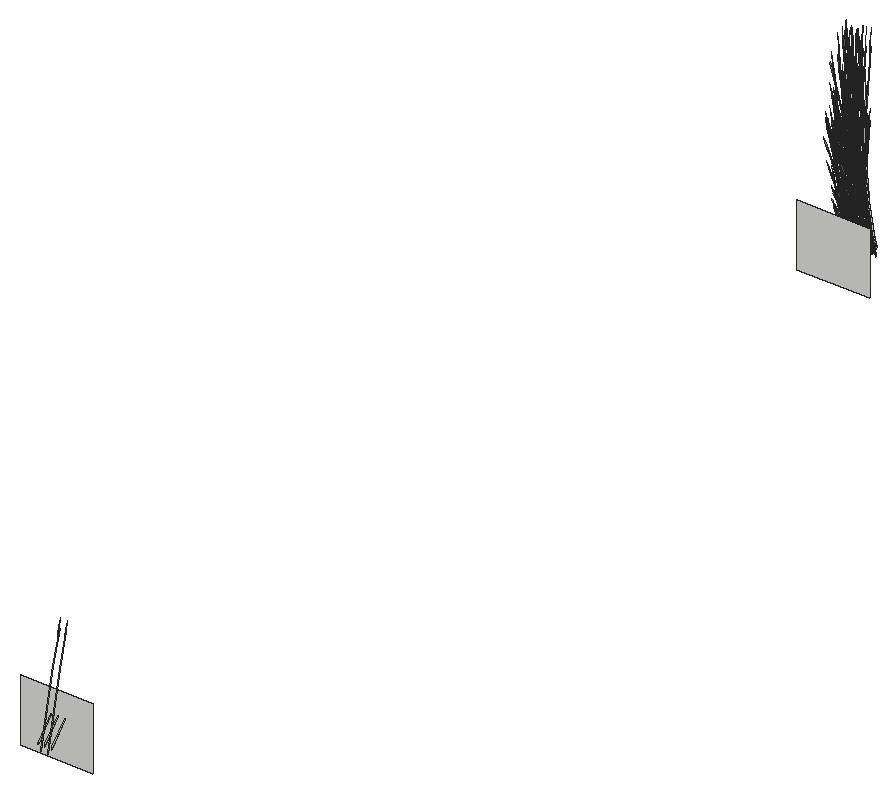
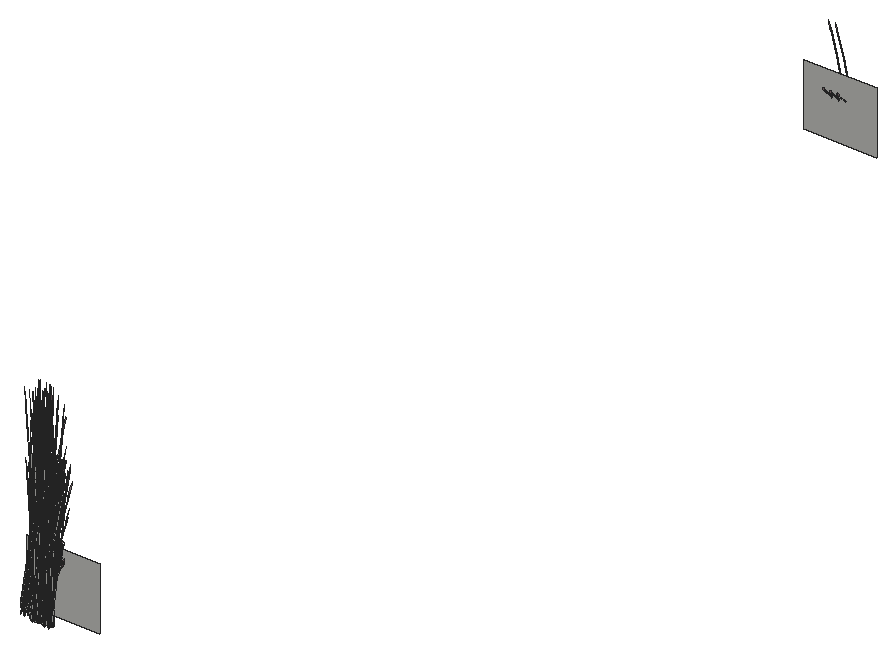
# SketchUp Ruby script. Lengths in inches.
U = 1.inch
M = Sketchup.active_model
def pt(a) = Geom::Point3d.new(a.map { |v| v * U })
def face(e, loops, mat)
  f = e.add_face(loops[0].map { |a| pt(a) })
  loops[1..].each { |l| e.add_face(l.map { |a| pt(a) }).erase! }
  f.material = f.back_material = mat if mat
  f
end
# faces: each face lists its corners as indices into pts; further lists are holes
def faces(e, pts, list, mat = nil) = list.each { |f| face(e, (f[0].is_a?(Array) ? f : [f]).map { |l| l.map { |i| pts[i] } }, mat) }
# xy, xz, yz: faces in a plane at the given z, y or x. An outline is a flat list of corners, or four numbers for a rectangle; further outlines are holes
def ring(l) = l.size == 4 ? [[l[0], l[1]], [l[2], l[1]], [l[2], l[3]], [l[0], l[3]]] : l.each_slice(2).to_a
def flat(e, list, mat, &to3) = list.each { |f| face(e, (f[0].is_a?(Array) ? f : [f]).map { |l| ring(l).map { |u, v| to3.(u, v) } }, mat) }
def xy(e, z, list, mat = nil) = flat(e, list, mat) { |x, y| [x, y, z] }
def xz(e, y, list, mat = nil) = flat(e, list, mat) { |x, z| [x, y, z] }
def yz(e, x, list, mat = nil) = flat(e, list, mat) { |y, z| [x, y, z] }
def lines(e, pts, list) = list.each { |a, b| e.add_line(pt(pts[a]), pt(pts[b])) }
# prism: a flat outline (further loops are holes) pulled along v
def prism(e, loops, v, mat = nil)
  f = face(e, loops, mat); d = Geom::Vector3d.new(v.map { |x| x * U })
  f.pushpull(f.normal.samedirection?(d) ? d.length : -d.length)
end
def box(e, o, s, mat = nil) = prism(e, [[o, [o[0] + s[0], o[1], o[2]], [o[0] + s[0], o[1] + s[1], o[2]], [o[0], o[1] + s[1], o[2]]]], [0, 0, s[2]], mat)
def at(x, y, z, deg = 0) = Geom::Transformation.translation(pt([x, y, z])) * Geom::Transformation.rotation(ORIGIN, Z_AXIS, deg.degrees)
def axes(o, x, y, z) = Geom::Transformation.new([*x, 0, *y, 0, *z, 0, *pt(o).to_a, 1])
def part(name) = M.definitions.add(name)
# library, detail: a bought-in or finely detailed component or shape, given as its bounding box
def library(name, o, s) = part(name).tap { |d| box(d.entities, o, s) }
def detail(e, o, s) = box(e.add_group.entities, o, s)
def put(e, d, t, mat = nil) = e.add_instance(d, t).tap { |i| i.material = mat if mat }
def group(e, t, mat = nil) = e.add_group.tap { |g| g.transformation = t; g.material = mat if mat }.entities
root = M.entities
M.materials.add("LightPink_Translucent").color = [144, 107, 117]
M.materials["LightPink_Translucent"].alpha = 0.75
c1 = part("blade")
p = [[2.15,0.21,22],[0,0.17,0],[0.09,0.45,0],[2.18,0.31,22],[2.29,0.31,22],[0.38,0.45,0],
  [2.48,0.24,33],[2.49,0.24,33],[2.48,0.22,33]]
faces(c1.entities,p,[[0,1,2,3],[4,5,2,3],[6,3,4,7],[8,0,3,6]])
c2 = part("seeds")
p = [[0.3,-0.1,1.38],[-0.01,-0.03,1.59],[-0.01,-0.03,0.03],[0.14,-0.07,-0.07],[0.29,-0.03,3],[0.15,0.01,3.11]]
faces(c2.entities,p,[[0,1,2,3],[1,0,4,5]],"LightPink_Translucent")
c3 = part("blade with seeds")
put(c3.entities,c1,at(0,0,0))
put(c3.entities,c2,axes([2.4,0.25,30.99],[1.5799,-0.05474,1.17369],[-0.12525,1.92788,0.29478],[-0.07173,-0.02425,1.56792]))
xz(root,361.54,[[333.57,618,354.57,636]])
xz(root,640.9,[[333.57,618,354.57,636]])
put(root,c3,axes([341.53,357.88,622.72],[0.04474,0.0751,1.74944],[0.36104,0.0295,-0.27667],[0.03631,0.16562,0.14031]))
put(root,c3,axes([345.44,357.89,622.72],[0.04474,0.0751,1.74944],[0.36104,0.0295,-0.27667],[0.03631,0.16562,0.14031]))
put(root,c3,axes([343.4,357.98,622.72],[0.04474,0.0751,1.74944],[0.36104,0.0295,-0.27667],[0.03631,0.16562,0.14031]))
put(root,c3,axes([344.86,357.17,621.36],[0.00775,-0.24075,1.54345],[0.34877,0.12716,0.21329],[-0.03022,0.25658,0.72882]))
put(root,c3,axes([342.82,357.26,621.36],[0.00775,-0.24075,1.54345],[0.34877,0.12716,0.21329],[-0.03022,0.25658,0.72882]))
put(root,c3,axes([343.9,649.42,623.6],[0.08068,0.14973,1.71376],[-0.3728,0.12606,0.13857],[-0.08426,-0.23506,0.73262]))
put(root,c3,axes([344.51,648.43,624.44],[-0.05398,-0.06539,1.74944],[-0.36026,0.04145,-0.27667],[-0.0575,-0.15639,0.14031]))
put(root,c3,axes([341,649.2,621.81],[-0.10032,0.0944,1.43002],[-0.30046,-0.16522,-0.30754],[0.05569,-0.20547,0.61141]))
put(root,c3,axes([342.08,649.2,621.91],[-0.10032,0.0944,1.43002],[-0.30046,-0.16522,-0.30754],[0.05569,-0.20547,0.61141]))
put(root,c3,axes([343.42,649.2,622.3],[-0.10032,0.0944,1.43002],[-0.30046,-0.16522,-0.30754],[0.05569,-0.20547,0.61141]))
put(root,c3,axes([345.35,649.2,622.32],[-0.10032,0.0944,1.43002],[-0.30046,-0.16522,-0.30754],[0.05569,-0.20547,0.61141]))
put(root,c3,axes([348.01,649.6,624.1],[0.08068,0.14973,1.71376],[-0.3728,0.12606,0.13857],[-0.08426,-0.23506,0.73262]))
put(root,c3,axes([342.96,649.53,624.6875],[-0.16845,-0.3792,-0.71045],[0.34676,-0.21133,0.08574],[-0.03939,-0.18322,1.00501]))
put(root,c3,axes([344.89,649.53,624.71],[-0.16845,-0.3792,-0.71045],[0.34676,-0.21133,0.08574],[-0.03939,-0.18322,1.00501]))
put(root,c3,axes([343.8,649.02,622.32],[-0.02137,0.15256,1.43002],[-0.31245,0.12771,-0.30754],[-0.07303,-0.19719,0.61141]))
put(root,c3,axes([342.67,648.6875,621.2],[-0.0592,0.0168,1.76342],[-0.32738,-0.18913,-0.26939],[0.00549,-0.15776,0.30037]))
put(root,c3,axes([344.6,648.6875,621.22],[-0.0592,0.0168,1.76342],[-0.32738,-0.18913,-0.26939],[0.00549,-0.15776,0.30037]))
put(root,c3,axes([347.91,649.2,622.82],[-0.02137,0.15256,1.43002],[-0.31245,0.12771,-0.30754],[-0.07303,-0.19719,0.61141]))
put(root,c3,axes([341.25,649.9,624.21],[0.00918,-0.43138,-0.71045],[0.38672,0.02897,0.08574],[0.04081,-0.18275,1.00501]))
put(root,c3,axes([342.33,649.9,624.3],[0.00918,-0.43138,-0.71045],[0.38672,0.02897,0.08574],[0.04081,-0.18275,1.00501]))
put(root,c3,axes([343.66,649.9,624.6875],[0.00918,-0.43138,-0.71045],[0.38672,0.02897,0.08574],[0.04081,-0.18275,1.00501]))
put(root,c3,axes([345.59,649.9,624.71],[0.00918,-0.43138,-0.71045],[0.38672,0.02897,0.08574],[0.04081,-0.18275,1.00501]))
put(root,c3,axes([341.79,649.23,623.9375],[-0.00341,-0.09282,1.74944],[-0.28775,-0.26825,-0.27667],[0.04449,-0.16261,0.14031]))
put(root,c3,axes([342.86,649.23,624.03],[-0.00341,-0.09282,1.74944],[-0.28775,-0.26825,-0.27667],[0.04449,-0.16261,0.14031]))
put(root,c3,axes([344.2,649.23,624.42],[-0.00341,-0.09282,1.74944],[-0.28775,-0.26825,-0.27667],[0.04449,-0.16261,0.14031]))
put(root,c3,axes([342.99,649.21,624.23],[0.1064,-0.35863,-0.35414],[0.31043,0.1046,0.4572],[-0.02846,-0.14439,0.87481]))
put(root,c3,axes([344.92,649.21,624.25],[0.1064,-0.35863,-0.35414],[0.31043,0.1046,0.4572],[-0.02846,-0.14439,0.87481]))
put(root,c3,axes([340.8125,649.68,623.1],[-0.06572,0.16029,1.71376],[-0.27569,-0.33172,0.13857],[0.12437,-0.20675,0.73262]))
put(root,c3,axes([341.89,649.68,623.19],[-0.06572,0.16029,1.71376],[-0.27569,-0.33172,0.13857],[0.12437,-0.20675,0.73262]))
put(root,c3,axes([343.23,649.68,623.58],[-0.06572,0.16029,1.71376],[-0.27569,-0.33172,0.13857],[0.12437,-0.20675,0.73262]))
put(root,c3,axes([342.79,648.89,624.03],[-0.03584,0.03562,1.77383],[-0.35118,-0.12018,-0.16761],[-0.01271,-0.15545,0.31391]))
put(root,c3,axes([344.12,648.89,624.42],[-0.03584,0.03562,1.77383],[-0.35118,-0.12018,-0.16761],[-0.01271,-0.15545,0.31391]))
put(root,c3,axes([346.06,648.89,624.43],[-0.03584,0.03562,1.77383],[-0.35118,-0.12018,-0.16761],[-0.01271,-0.15545,0.31391]))
put(root,c3,axes([342.83,649.45,624.39],[-0.34695,-0.11691,-0.51099],[0.11892,-0.40083,-0.3958],[-0.03181,-0.16138,0.97773]))
put(root,c3,axes([344.77,649.45,624.41],[-0.34695,-0.11691,-0.51099],[0.11892,-0.40083,-0.3958],[-0.03181,-0.16138,0.97773]))
put(root,c3,axes([341.71,648.45,622.08],[0.04528,0.27194,1.1486],[-0.25117,-0.15062,0.84392],[0.02703,-0.13924,0.25299]))
put(root,c3,axes([343.05,648.45,622.47],[0.04528,0.27194,1.1486],[-0.25117,-0.15062,0.84392],[0.02703,-0.13924,0.25299]))
put(root,c3,axes([344.98,648.45,622.49],[0.04528,0.27194,1.1486],[-0.25117,-0.15062,0.84392],[0.02703,-0.13924,0.25299]))
put(root,c3,axes([341.17,649.76,623.9],[-0.25266,-0.31335,-0.51099],[0.2669,-0.27442,-0.3958],[0.03844,-0.15921,0.97773]))
put(root,c3,axes([342.25,649.76,624],[-0.25266,-0.31335,-0.51099],[0.2669,-0.27442,-0.3958],[0.03844,-0.15921,0.97773]))
put(root,c3,axes([343.58,649.76,624.39],[-0.25266,-0.31335,-0.51099],[0.2669,-0.27442,-0.3958],[0.03844,-0.15921,0.97773]))
put(root,c3,axes([345.52,649.76,624.41],[-0.25266,-0.31335,-0.51099],[0.2669,-0.27442,-0.3958],[0.03844,-0.15921,0.97773]))
put(root,c3,axes([344.15,648.21,624.43],[-0.00658,0.0559,1.77383],[-0.32474,0.20287,-0.16761],[-0.09556,-0.1037,0.31391]))
put(root,c3,axes([344.07,649.2,624.82],[0.39316,-0.11987,0.53763],[0.06823,0.47021,0.4433],[-0.09247,-0.13858,1.11249]))
put(root,c3,axes([348.26,648.39,624.93],[-0.00658,0.0559,1.77383],[-0.32474,0.20287,-0.16761],[-0.09556,-0.1037,0.31391]))
put(root,c3,axes([341.69,649.29,624.05],[0.34777,0.12192,0.48003],[-0.11892,0.40083,0.3958],[-0.0209,-0.15763,0.9933]))
put(root,c3,axes([343.03,649.29,624.44],[0.34777,0.12192,0.48003],[-0.11892,0.40083,0.3958],[-0.0209,-0.15763,0.9933]))
put(root,c3,axes([344.96,649.29,624.46],[0.34777,0.12192,0.48003],[-0.11892,0.40083,0.3958],[-0.0209,-0.15763,0.9933]))
put(root,c3,axes([343.13,649.43,624.74],[-0.34538,0.21713,-0.1216],[-0.16972,-0.38536,-0.67495],[-0.04557,-0.16239,1.02557]))
put(root,c3,axes([345.0625,649.43,624.76],[-0.34538,0.21713,-0.1216],[-0.16972,-0.38536,-0.67495],[-0.04557,-0.16239,1.02557]))
put(root,c3,axes([342.51,649.92,624.35],[-0.3879,-0.02311,-0.1216],[0.0106,-0.43749,-0.67495],[0.02694,-0.1685,1.02557]))
put(root,c3,axes([343.85,649.92,624.74],[-0.3879,-0.02311,-0.1216],[0.0106,-0.43749,-0.67495],[0.02694,-0.1685,1.02557]))
put(root,c3,axes([345.78,649.92,624.76],[-0.3879,-0.02311,-0.1216],[0.0106,-0.43749,-0.67495],[0.02694,-0.1685,1.02557]))
put(root,c3,axes([341.41,649.64,623.75],[0.23881,-0.24554,-0.35414],[0.22606,0.28036,0.4572],[0.0344,-0.14245,0.87481]))
put(root,c3,axes([342.49,649.64,623.84],[0.23881,-0.24554,-0.35414],[0.22606,0.28036,0.4572],[0.0344,-0.14245,0.87481]))
put(root,c3,axes([343.82,649.64,624.23],[0.23881,-0.24554,-0.35414],[0.22606,0.28036,0.4572],[0.0344,-0.14245,0.87481]))
put(root,c3,axes([345.75,649.64,624.25],[0.23881,-0.24554,-0.35414],[0.22606,0.28036,0.4572],[0.0344,-0.14245,0.87481]))
put(root,c3,axes([343.6875,648.78,622.49],[0.18411,0.16231,1.1486],[-0.26813,0.09757,0.84392],[-0.05737,-0.12474,0.25299]))
put(root,c3,axes([341.79,649.26,624.05],[0.26007,-0.1585,0.0643],[0.12729,0.28902,0.50621],[-0.02512,-0.1274,0.77189]))
put(root,c3,axes([343.12,649.26,624.4375],[0.26007,-0.1585,0.0643],[0.12729,0.28902,0.50621],[-0.02512,-0.1274,0.77189]))
put(root,c3,axes([345.06,649.26,624.46],[0.26007,-0.1585,0.0643],[0.12729,0.28902,0.50621],[-0.02512,-0.1274,0.77189]))
put(root,c3,axes([344.13,649.64,624.71],[-0.30095,-0.22541,-0.71045],[0.21388,-0.395,0.08574],[-0.10904,-0.13459,1.00501]))
put(root,c3,axes([344.03,649.34,624.25],[-0.05451,-0.37564,-0.35414],[0.31161,-0.09919,0.4572],[-0.0837,-0.10765,0.87481]))
put(root,c3,axes([348.25,649.82,625.21],[-0.30095,-0.22541,-0.71045],[0.21388,-0.395,0.08574],[-0.10904,-0.13459,1.00501]))
put(root,c3,axes([348.14,649.52,624.75],[-0.05451,-0.37564,-0.35414],[0.31161,-0.09919,0.4572],[-0.0837,-0.10765,0.87481]))
put(root,c3,axes([344.16,649.3,624.46],[0.16041,-0.29625,0.0643],[0.22843,0.17248,0.50621],[-0.07385,-0.09498,0.77189]))
put(root,c3,axes([343.54,649.27,621.22],[-0.03419,0.06144,1.76342],[-0.3455,0.13246,-0.26939],[-0.08346,-0.12049,0.30037]))
put(root,c3,axes([342.18,650.95,621.81],[-0.14494,-0.47823,-0.69835],[0.41752,-0.17223,-0.18329],[-0.01602,-0.16194,1.54149]))
put(root,c3,axes([344.11,650.95,621.82],[-0.14494,-0.47823,-0.69835],[0.41752,-0.17223,-0.18329],[-0.01602,-0.16194,1.54149]))
put(root,c3,axes([341.71,649.49,620.72],[-0.05283,-0.03674,1.76342],[-0.13569,-0.41045,-0.26939],[0.09154,-0.11138,0.30037]))
put(root,c3,axes([342.78,649.49,620.81],[-0.05283,-0.03674,1.76342],[-0.13569,-0.41045,-0.26939],[0.09154,-0.11138,0.30037]))
put(root,c3,axes([344.12,649.49,621.2],[-0.05283,-0.03674,1.76342],[-0.13569,-0.41045,-0.26939],[0.09154,-0.11138,0.30037]))
put(root,c3,axes([347.66,649.45,621.72],[-0.03419,0.06144,1.76342],[-0.3455,0.13246,-0.26939],[-0.08346,-0.12049,0.30037]))
put(root,c3,axes([343.03,649.59,624.76],[-0.1064,0.35863,0.35414],[-0.31043,-0.1046,-0.4572],[-0.02846,-0.14439,0.87481]))
put(root,c3,axes([344.96,649.59,624.78],[-0.1064,0.35863,0.35414],[-0.31043,-0.1046,-0.4572],[-0.02846,-0.14439,0.87481]))
put(root,c3,axes([347.47,650.06,624.1],[0.1311,0.08035,1.71376],[-0.27131,0.33708,0.13857],[-0.16909,-0.15206,0.73262]))
put(root,c3,axes([343.99,649.65,624.41],[-0.34827,0.11086,-0.51099],[-0.06092,-0.41983,-0.3958],[-0.09354,-0.12031,0.97773]))
put(root,c3,axes([341.41,649.74,623.96],[0.25132,0.3182,0.48003],[-0.2669,0.27442,0.3958],[0.04636,-0.14929,0.9933]))
put(root,c3,axes([342.48,649.74,624.05],[0.25132,0.3182,0.48003],[-0.2669,0.27442,0.3958],[0.04636,-0.14929,0.9933]))
put(root,c3,axes([343.82,649.74,624.44],[0.25132,0.3182,0.48003],[-0.2669,0.27442,0.3958],[0.04636,-0.14929,0.9933]))
put(root,c3,axes([344.24,649.27,625.16],[-0.23555,0.44708,-0.13619],[-0.34112,-0.25757,-0.75594],[-0.11858,-0.12631,1.14864]))
put(root,c3,axes([341.5,649.77,623.95],[0.29004,0.02173,0.0643],[-0.00795,0.32812,0.50621],[0.03035,-0.12569,0.77189]))
put(root,c3,axes([342.58,649.77,624.05],[0.29004,0.02173,0.0643],[-0.00795,0.32812,0.50621],[0.03035,-0.12569,0.77189]))
put(root,c3,axes([343.91,649.77,624.4375],[0.29004,0.02173,0.0643],[-0.00795,0.32812,0.50621],[0.03035,-0.12569,0.77189]))
put(root,c3,axes([345.84,649.77,624.46],[0.29004,0.02173,0.0643],[-0.00795,0.32812,0.50621],[0.03035,-0.12569,0.77189]))
put(root,c3,axes([342.36,649.99,624.37],[-0.23881,0.24554,0.35414],[-0.22606,-0.28036,-0.4572],[0.0344,-0.14245,0.87481]))
put(root,c3,axes([343.7,649.99,624.76],[-0.23881,0.24554,0.35414],[-0.22606,-0.28036,-0.4572],[0.0344,-0.14245,0.87481]))
put(root,c3,axes([345.63,649.99,624.78],[-0.23881,0.24554,0.35414],[-0.22606,-0.28036,-0.4572],[0.0344,-0.14245,0.87481]))
put(root,c3,axes([348.11,649.83,624.91],[-0.34827,0.11086,-0.51099],[-0.06092,-0.41983,-0.3958],[-0.09354,-0.12031,0.97773]))
put(root,c3,axes([348.67,650.3,623.57],[0.1311,0.08035,1.71376],[-0.27131,0.33708,0.13857],[-0.16909,-0.15206,0.73262]))
put(root,c3,axes([348.35,649.45,625.66],[-0.23555,0.44708,-0.13619],[-0.34112,-0.25757,-0.75594],[-0.11858,-0.12631,1.14864]))
put(root,c3,axes([341.7,650.65,624.21],[0.18436,-0.36797,-0.71045],[0.32306,0.26151,0.08574],[0.11008,-0.13332,1.00501]))
put(root,c3,axes([342.78,650.65,624.3],[0.18436,-0.36797,-0.71045],[0.32306,0.26151,0.08574],[0.11008,-0.13332,1.00501]))
put(root,c3,axes([344.12,650.65,624.6875],[0.18436,-0.36797,-0.71045],[0.32306,0.26151,0.08574],[0.11008,-0.13332,1.00501]))
put(root,c3,axes([340.79,649.58,621.69],[-0.22066,-0.46731,0],[0.36918,-0.26061,-0.51607],[0.08408,-0.05936,1.63711]))
put(root,c3,axes([342.125,649.58,622.08],[-0.22066,-0.46731,0],[0.36918,-0.26061,-0.51607],[0.08408,-0.05936,1.63711]))
put(root,c3,axes([344.06,649.58,622.1],[-0.22066,-0.46731,0],[0.36918,-0.26061,-0.51607],[0.08408,-0.05936,1.63711]))
put(root,c3,axes([341.69,650.48,623.9],[-0.09067,-0.42583,-0.51099],[0.34336,-0.07449,-0.3958],[0.0984,-0.11438,0.97773]))
put(root,c3,axes([342.77,650.48,624],[-0.09067,-0.42583,-0.51099],[0.34336,-0.07449,-0.3958],[0.0984,-0.11438,0.97773]))
put(root,c3,axes([344.11,650.48,624.39],[-0.09067,-0.42583,-0.51099],[0.34336,-0.07449,-0.3958],[0.0984,-0.11438,0.97773]))
put(root,c3,axes([342.61,649.02,621.84],[-0.2439,0.26754,-0.03893],[-0.22348,-0.29302,-0.17649],[-0.01573,-0.08303,0.58215]))
put(root,c3,axes([344.54,649.02,621.85],[-0.2439,0.26754,-0.03893],[-0.22348,-0.29302,-0.17649],[-0.01573,-0.08303,0.58215]))
put(root,c3,axes([341.86,650.78,624.26],[-0.32648,-0.25715,-0.1216],[0.18809,-0.3724,-0.67495],[0.09224,-0.12945,1.02557]))
put(root,c3,axes([342.93,650.78,624.35],[-0.32648,-0.25715,-0.1216],[0.18809,-0.3724,-0.67495],[0.09224,-0.12945,1.02557]))
put(root,c3,axes([344.27,650.78,624.74],[-0.32648,-0.25715,-0.1216],[0.18809,-0.3724,-0.67495],[0.09224,-0.12945,1.02557]))
put(root,c3,axes([347.45,649.32,624.94],[-0.07594,-0.00329,1.74944],[-0.24177,0.32918,-0.27667],[-0.129,-0.06726,0.14031]))
put(root,c3,axes([344.85,652.1875,623.05],[0.305,0.18805,1.51261],[-0.29879,0.40513,0.59816],[-0.13384,-0.24012,1.26806]))
put(root,c3,axes([344.21,649.65,624.78],[0.05451,0.37564,0.35414],[-0.31161,0.09919,-0.4572],[-0.0837,-0.10765,0.87481]))
put(root,c3,axes([343.26,650.89,621.74],[0,-0.46636,-0.49651],[0.39487,0,0],[0,-0.10622,1.57504]))
put(root,c3,axes([340.01,649.51,621.24],[0.33032,-0.23318,-0.49651],[0.19744,0.41812,0],[0.07523,-0.05311,1.57504]))
put(root,c3,axes([341.09,649.51,621.33],[0.33032,-0.23318,-0.49651],[0.19744,0.41812,0],[0.07523,-0.05311,1.57504]))
put(root,c3,axes([342.42,649.51,621.72],[0.33032,-0.23318,-0.49651],[0.19744,0.41812,0],[0.07523,-0.05311,1.57504]))
put(root,c3,axes([344.36,649.51,621.74],[0.33032,-0.23318,-0.49651],[0.19744,0.41812,0],[0.07523,-0.05311,1.57504]))
put(root,c3,axes([341.97,650.3125,621.81],[-0.12609,-0.01381,1.43002],[-0.12917,-0.37055,-0.30754],[0.1549,-0.10482,0.61141]))
put(root,c3,axes([343.05,650.3125,621.91],[-0.12609,-0.01381,1.43002],[-0.12917,-0.37055,-0.30754],[0.1549,-0.10482,0.61141]))
put(root,c3,axes([342.66,650.67,623.93],[-0.0461,-0.00354,1.77383],[-0.19143,-0.37951,-0.16761],[0.07688,-0.12478,0.31391]))
put(root,c3,axes([343.74,650.67,624.03],[-0.0461,-0.00354,1.77383],[-0.19143,-0.37951,-0.16761],[0.07688,-0.12478,0.31391]))
put(root,c3,axes([345.07,650.67,624.42],[-0.0461,-0.00354,1.77383],[-0.19143,-0.37951,-0.16761],[0.07688,-0.12478,0.31391]))
put(root,c3,axes([348.64,649.5625,624.41],[-0.07594,-0.00329,1.74944],[-0.24177,0.32918,-0.27667],[-0.129,-0.06726,0.14031]))
put(root,c3,axes([340.4,650.46,621.28],[0.23773,-0.35053,-0.62353],[0.29532,0.31785,-0.16365],[0.09526,-0.08744,1.37633]))
put(root,c3,axes([341.48,650.46,621.375],[0.23773,-0.35053,-0.62353],[0.29532,0.31785,-0.16365],[0.09526,-0.08744,1.37633]))
put(root,c3,axes([342.81,650.46,621.77],[0.23773,-0.35053,-0.62353],[0.29532,0.31785,-0.16365],[0.09526,-0.08744,1.37633]))
put(root,c3,axes([342.12,649.63,621.99],[-0.11756,0.2374,1.1486],[-0.10105,-0.31895,0.84392],[0.09709,-0.07992,0.25299]))
put(root,c3,axes([343.19,649.63,622.08],[-0.11756,0.2374,1.1486],[-0.10105,-0.31895,0.84392],[0.09709,-0.07992,0.25299]))
put(root,c3,axes([344.53,649.63,622.47],[-0.11756,0.2374,1.1486],[-0.10105,-0.31895,0.84392],[0.09709,-0.07992,0.25299]))
put(root,c3,axes([347.39,650.07,625.32],[0.29147,-0.34417,0.53763],[0.25138,0.3655,0.4433],[-0.13675,-0.06349,1.11249]))
put(root,c3,axes([341.95,650.52,623.75],[0.30722,-0.06665,-0.35414],[0.08112,0.381,0.4572],[0.08804,-0.10234,0.87481]))
put(root,c3,axes([343.03,650.52,623.84],[0.30722,-0.06665,-0.35414],[0.08112,0.381,0.4572],[0.08804,-0.10234,0.87481]))
put(root,c3,axes([344.36,650.52,624.23],[0.30722,-0.06665,-0.35414],[0.08112,0.381,0.4572],[0.08804,-0.10234,0.87481]))
put(root,c3,axes([343.41,649.89,624.46],[0.01777,-0.35463,0.0643],[0.26836,0.00972,0.50621],[-0.1028,-0.03711,0.77189]))
put(root,c3,axes([348.59,650.31,624.78],[0.29147,-0.34417,0.53763],[0.25138,0.3655,0.4433],[-0.13675,-0.06349,1.11249]))
put(root,c3,axes([342.4,651.08,621.92],[0.17124,-0.42022,-0.44739],[0.35581,0.20224,0.21531],[0,-0.09687,1.43643]))
put(root,c3,axes([344.33,651.08,621.9375],[0.17124,-0.42022,-0.44739],[0.35581,0.20224,0.21531],[0,-0.09687,1.43643]))
put(root,c3,axes([341.22,650.87,621.98],[-0.04113,-0.53214,-0.29095],[0.42835,-0.03218,-0.50002],[0.07543,-0.07088,1.59708]))
put(root,c3,axes([342.56,650.87,622.375],[-0.04113,-0.53214,-0.29095],[0.42835,-0.03218,-0.50002],[0.07543,-0.07088,1.59708]))
put(root,c3,axes([344.49,650.87,622.39],[-0.04113,-0.53214,-0.29095],[0.42835,-0.03218,-0.50002],[0.07543,-0.07088,1.59708]))
put(root,c3,axes([341.5,650.9,621.74],[0.24637,-0.29097,-0.30978],[0.24637,0.29097,0.30978],[0,-0.09372,1.38974]))
put(root,c3,axes([343.43,650.9,621.75],[0.24637,-0.29097,-0.30978],[0.24637,0.29097,0.30978],[0,-0.09372,1.38974]))
put(root,c3,axes([347.53,650.07,624.96],[0.01777,-0.35463,0.0643],[0.26836,0.00972,0.50621],[-0.1028,-0.03711,0.77189]))
put(root,c3,axes([343.33,649.5,621.85],[-0.10181,0.3808,-0.03893],[-0.31336,-0.11714,-0.17649],[-0.04758,-0.06228,0.58215]))
put(root,c3,axes([341.7,650.75,624.28],[-0.30722,0.06665,0.35414],[-0.08112,-0.381,-0.4572],[0.08804,-0.10234,0.87481]))
put(root,c3,axes([342.78,650.75,624.37],[-0.30722,0.06665,0.35414],[-0.08112,-0.381,-0.4572],[0.08804,-0.10234,0.87481]))
put(root,c3,axes([344.11,650.75,624.76],[-0.30722,0.06665,0.35414],[-0.08112,-0.381,-0.4572],[0.08804,-0.10234,0.87481]))
put(root,c3,axes([342.36,651.43,622.375],[-0.39748,-0.22252,-0.29095],[0.19139,-0.46966,-0.50002],[-0.01249,-0.11531,1.59708]))
put(root,c3,axes([344.29,651.43,622.39],[-0.39748,-0.22252,-0.29095],[0.19139,-0.46966,-0.50002],[-0.01249,-0.11531,1.59708]))
put(root,c3,axes([347.42,650.18,624.75],[-0.20082,-0.29199,-0.35414],[0.2293,-0.2764,0.4572],[-0.1165,-0.04206,0.87481]))
put(root,c3,axes([343.16,651.24,622.1],[-0.44133,0,0],[0,-0.52122,-0.51607],[0,-0.11871,1.63711]))
put(root,c3,axes([347.44,649.68,622.35],[-0.10181,0.3808,-0.03893],[-0.31336,-0.11714,-0.17649],[-0.04758,-0.06228,0.58215]))
put(root,c3,axes([340.09,649.69,621.25],[0.32928,0.11539,-0.30978],[-0.08291,0.40636,0.30978],[0.06638,-0.04686,1.38974]))
put(root,c3,axes([341.17,649.69,621.35],[0.32928,0.11539,-0.30978],[-0.08291,0.40636,0.30978],[0.06638,-0.04686,1.38974]))
put(root,c3,axes([342.5,649.69,621.74],[0.32928,0.11539,-0.30978],[-0.08291,0.40636,0.30978],[0.06638,-0.04686,1.38974]))
put(root,c3,axes([344.43,649.69,621.75],[0.32928,0.11539,-0.30978],[-0.08291,0.40636,0.30978],[0.06638,-0.04686,1.38974]))
put(root,c3,axes([347.28,651.42,622.6],[-0.44133,0,0],[0,-0.52122,-0.51607],[0,-0.11871,1.63711]))
put(root,c3,axes([348.62,650.42,624.22],[-0.20082,-0.29199,-0.35414],[0.2293,-0.2764,0.4572],[-0.1165,-0.04206,0.87481]))
put(root,c3,axes([347.35,650.49,622.82],[0.06891,0.12984,1.43002],[-0.15879,0.35293,-0.30754],[-0.16304,-0.08436,0.61141]))
put(root,c3,axes([347.64,650.375,625.21],[-0.35281,-0.01123,-0.71045],[0.0237,-0.47284,0.08574],[-0.14947,-0.0499,1.00501]))
put(root,c3,axes([341.98,650.6875,623.95],[0.2423,0.19613,0.0643],[-0.14107,0.2793,0.50621],[0.07768,-0.0903,0.77189]))
put(root,c3,axes([343.05,650.6875,624.05],[0.2423,0.19613,0.0643],[-0.14107,0.2793,0.50621],[0.07768,-0.0903,0.77189]))
put(root,c3,axes([344.39,650.6875,624.4375],[0.2423,0.19613,0.0643],[-0.14107,0.2793,0.50621],[0.07768,-0.0903,0.77189]))
put(root,c3,axes([341.91,650.61,623.96],[0.08753,0.42921,0.48003],[-0.34336,0.07449,0.3958],[0.1012,-0.10094,0.9933]))
put(root,c3,axes([342.99,650.61,624.05],[0.08753,0.42921,0.48003],[-0.34336,0.07449,0.3958],[0.1012,-0.10094,0.9933]))
put(root,c3,axes([344.32,650.61,624.44],[0.08753,0.42921,0.48003],[-0.34336,0.07449,0.3958],[0.1012,-0.10094,0.9933]))
put(root,c3,axes([342.83,651.125,623.9375],[0.04898,-0.07104,1.74944],[-0.06269,-0.43574,-0.27667],[0.12289,-0.08262,0.14031]))
put(root,c3,axes([343.91,651.125,624.03],[0.04898,-0.07104,1.74944],[-0.06269,-0.43574,-0.27667],[0.12289,-0.08262,0.14031]))
put(root,c3,axes([348.54,650.73,622.28],[0.06891,0.12984,1.43002],[-0.15879,0.35293,-0.30754],[-0.16304,-0.08436,0.61141]))
put(root,c3,axes([343.5,651.1,622.06],[-0.32829,0.39208,0.30756],[-0.32849,-0.38796,-0.36492],[-0.01146,-0.11134,1.64885]))
put(root,c3,axes([348.83,650.61,624.67],[-0.35281,-0.01123,-0.71045],[0.0237,-0.47284,0.08574],[-0.14947,-0.0499,1.00501]))
put(root,c3,axes([341.28,651.29,621.75],[0.39767,0.22603,0.24065],[-0.19139,0.46966,0.50002],[0,-0.10827,1.60543]))
put(root,c3,axes([342.61,651.29,622.14],[0.39767,0.22603,0.24065],[-0.19139,0.46966,0.50002],[0,-0.10827,1.60543]))
put(root,c3,axes([344.55,651.29,622.16],[0.39767,0.22603,0.24065],[-0.19139,0.46966,0.50002],[0,-0.10827,1.60543]))
put(root,c3,axes([344.39,651.92,622.16],[0.09355,-0.55261,-0.23429],[0.44354,0.09633,0.51271],[-0.0775,-0.07631,1.5644]))
put(root,c3,axes([347.16,649.6,624.93],[0.02617,0.04654,1.77383],[-0.12614,0.41836,-0.16761],[-0.12775,0.00303,0.31391]))
put(root,c3,axes([343.59,650.15,624.78],[0.20082,0.29199,0.35414],[-0.2293,0.2764,-0.4572],[-0.1165,-0.04206,0.87481]))
put(root,c3,axes([347.52,650.47,624.91],[-0.25628,0.30892,-0.51099],[-0.22444,-0.32634,-0.3958],[-0.13021,-0.047,0.97773]))
put(root,c3,axes([341.15,650.97,622.04],[-0.38326,0.02879,0.44739],[-0.03466,-0.47788,-0.21531],[0.06861,-0.04843,1.43643]))
put(root,c3,axes([342.48,650.97,622.43],[-0.38326,0.02879,0.44739],[-0.03466,-0.47788,-0.21531],[0.06861,-0.04843,1.43643]))
put(root,c3,axes([344.42,650.97,622.44],[-0.38326,0.02879,0.44739],[-0.03466,-0.47788,-0.21531],[0.06861,-0.04843,1.43643]))
put(root,c3,axes([347.71,650.33,625.28],[0.20082,0.29199,0.35414],[-0.2293,0.2764,-0.4572],[-0.1165,-0.04206,0.87481]))
put(root,c3,axes([348.35,649.84,624.4],[0.02617,0.04654,1.77383],[-0.12614,0.41836,-0.16761],[-0.12775,0.00303,0.31391]))
put(root,c3,axes([343.43,651.32,622.2],[0,0.46636,0.49651],[-0.39487,0,0],[0,-0.10622,1.57504]))
put(root,c3,axes([346.94,650.88,622.99],[0.22533,-0.03337,1.1486],[-0.14293,0.29403,0.84392],[-0.11135,-0.04411,0.25299]))
put(root,c3,axes([341.87,651.79,624.26],[-0.17758,-0.42229,-0.1216],[0.31518,-0.20752,-0.67495],[0.13282,-0.05572,1.02557]))
put(root,c3,axes([342.95,651.79,624.35],[-0.17758,-0.42229,-0.1216],[0.31518,-0.20752,-0.67495],[0.13282,-0.05572,1.02557]))
put(root,c3,axes([344.28,651.79,624.74],[-0.17758,-0.42229,-0.1216],[0.31518,-0.20752,-0.67495],[0.13282,-0.05572,1.02557]))
put(root,c3,axes([341.85,651.42,623.9],[0.09562,-0.42421,-0.51099],[0.32782,0.1454,-0.3958],[0.13199,-0.0389,0.97773]))
put(root,c3,axes([342.93,651.42,624],[0.09562,-0.42421,-0.51099],[0.32782,0.1454,-0.3958],[0.13199,-0.0389,0.97773]))
put(root,c3,axes([341.34,649.7,621.6],[0.22066,-0.46731,0],[0.36918,0.26061,-0.51607],[0.08408,0.05936,1.63711]))
put(root,c3,axes([342.41,649.7,621.69],[0.22066,-0.46731,0],[0.36918,0.26061,-0.51607],[0.08408,0.05936,1.63711]))
put(root,c3,axes([343.75,649.7,622.08],[0.22066,-0.46731,0],[0.36918,0.26061,-0.51607],[0.08408,0.05936,1.63711]))
put(root,c3,axes([344.36,651.7,621.9375],[-0.21202,-0.39143,-0.44739],[0.32115,-0.27564,0.21531],[-0.06861,-0.04843,1.43643]))
put(root,c3,axes([342.47,651.14,622.07],[0.15345,0.52148,0.45755],[-0.43845,0.18134,0.17955],[0.00536,-0.09582,1.58856]))
put(root,c3,axes([344.4,651.14,622.09],[0.15345,0.52148,0.45755],[-0.43845,0.18134,0.17955],[0.00536,-0.09582,1.58856]))
put(root,c3,axes([347.65,650.15,625.26],[-0.0189,0.47427,-0.1216],[-0.35781,-0.01296,-0.67495],[-0.13781,-0.03295,1.02557]))
put(root,c3,axes([348.71,650.71,624.37],[-0.25628,0.30892,-0.51099],[-0.22444,-0.32634,-0.3958],[-0.13021,-0.047,0.97773]))
